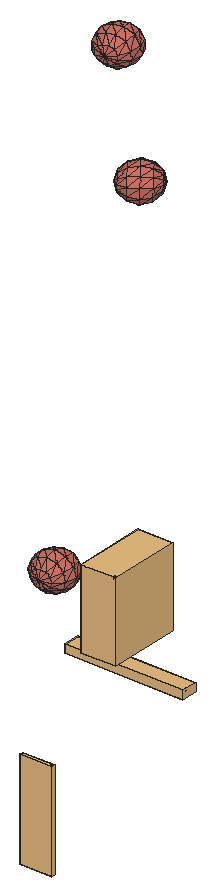
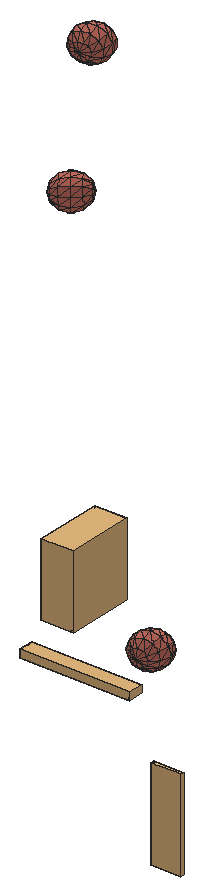
# SketchUp Ruby script. Lengths in inches.
U = 1.inch
M = Sketchup.active_model
def pt(a) = Geom::Point3d.new(a.map { |v| v * U })
def face(e, loops, mat)
  f = e.add_face(loops[0].map { |a| pt(a) })
  loops[1..].each { |l| e.add_face(l.map { |a| pt(a) }).erase! }
  f.material = f.back_material = mat if mat
  f
end
# faces: each face lists its corners as indices into pts; further lists are holes
def faces(e, pts, list, mat = nil) = list.each { |f| face(e, (f[0].is_a?(Array) ? f : [f]).map { |l| l.map { |i| pts[i] } }, mat) }
# xy, xz, yz: faces in a plane at the given z, y or x. An outline is a flat list of corners, or four numbers for a rectangle; further outlines are holes
def ring(l) = l.size == 4 ? [[l[0], l[1]], [l[2], l[1]], [l[2], l[3]], [l[0], l[3]]] : l.each_slice(2).to_a
def flat(e, list, mat, &to3) = list.each { |f| face(e, (f[0].is_a?(Array) ? f : [f]).map { |l| ring(l).map { |u, v| to3.(u, v) } }, mat) }
def xy(e, z, list, mat = nil) = flat(e, list, mat) { |x, y| [x, y, z] }
def xz(e, y, list, mat = nil) = flat(e, list, mat) { |x, z| [x, y, z] }
def yz(e, x, list, mat = nil) = flat(e, list, mat) { |y, z| [x, y, z] }
def lines(e, pts, list) = list.each { |a, b| e.add_line(pt(pts[a]), pt(pts[b])) }
# prism: a flat outline (further loops are holes) pulled along v
def prism(e, loops, v, mat = nil)
  f = face(e, loops, mat); d = Geom::Vector3d.new(v.map { |x| x * U })
  f.pushpull(f.normal.samedirection?(d) ? d.length : -d.length)
end
def box(e, o, s, mat = nil) = prism(e, [[o, [o[0] + s[0], o[1], o[2]], [o[0] + s[0], o[1] + s[1], o[2]], [o[0], o[1] + s[1], o[2]]]], [0, 0, s[2]], mat)
def at(x, y, z, deg = 0) = Geom::Transformation.translation(pt([x, y, z])) * Geom::Transformation.rotation(ORIGIN, Z_AXIS, deg.degrees)
def axes(o, x, y, z) = Geom::Transformation.new([*x, 0, *y, 0, *z, 0, *pt(o).to_a, 1])
def part(name) = M.definitions.add(name)
# library, detail: a bought-in or finely detailed component or shape, given as its bounding box
def library(name, o, s) = part(name).tap { |d| box(d.entities, o, s) }
def detail(e, o, s) = box(e.add_group.entities, o, s)
def put(e, d, t, mat = nil) = e.add_instance(d, t).tap { |i| i.material = mat if mat }
def group(e, t, mat = nil) = e.add_group.tap { |g| g.transformation = t; g.material = mat if mat }.entities
root = M.entities
M.materials.add("green").color = [174, 139, 102]
M.materials.add("vio").color = [206, 114, 100]
c1 = part("3DGeom~226_Defintion")
p = [[20.8,-212.46,-433.01],[-229.2,0,-445.02],[24.02,0,-500],[268.02,-184,-362.99],[268.02,-184,-362.99],[270.8,0,-421],
  [-231.98,184,-387.01],[20.8,212.47,-433.01],[270.8,0,-421],[-231.98,-184,-387.01],[-421,0,-270.8],[-422.61,106.23,-237.31],
  [-422.61,106.23,-237.31],[12.01,-368,-250],[260.4,-318.7,-204.5],[260.4,-318.7,-204.5],[268.02,-184,-362.99],[270.8,0,-421],
  [268.02,184,-362.99],[-239.6,318.7,-228.52],[268.02,184,-362.99],[12.01,368,-250],[-239.6,318.7,-228.52],[12.01,368,-250],
  [443.41,-106.23,-195.7],[268.02,-184,-362.99],[270.8,0,-421],[445.02,0,-229.2],[268.02,184,-362.99],[-239.6,-318.7,-228.52],
  [-239.6,-318.7,-228.52],[-422.61,-106.23,-237.31],[-231.98,-184,-387.01],[-422.61,-106.23,-237.31],[-231.98,184,-387.01],[-422.61,106.23,-237.31],
  [-427.01,184,-145.8],[-231.98,184,-387.01],[-239.6,318.7,-228.52],[439.02,-184,-104.2],[260.4,-318.7,-204.5],[443.41,106.23,-195.7],
  [260.4,318.7,-204.5],[268.02,184,-362.99],[12.01,368,-250],[260.4,318.7,-204.5],[-421,0,-270.8],[-422.61,-106.23,-237.31],
  [-500,0,-24.02],[-421,0,-270.8],[0,-424.93,0],[-239.6,-318.7,-228.52],[12.01,-368,-250],[250,-368,12.01],
  [12.01,-368,-250],[250,-368,12.01],[12.01,-368,-250],[260.4,-318.7,-204.5],[12.01,368,-250],[-239.6,318.7,-228.52],
  [-250,368,-12.01],[260.4,318.7,-204.5],[0,424.93,0],[-239.6,-318.7,-228.52],[-427.01,-184,-145.8],[-422.61,-106.23,-237.31],
  [-422.61,-106.23,-237.31],[500,0,24.02],[-250,-368,-12.01],[-239.6,-318.7,-228.52],[-250,-368,-12.01],[-239.6,-318.7,-228.52],
  [-239.6,318.7,-228.52],[-433.01,212.47,-20.8],[-239.6,318.7,-228.52],[-250,368,-12.01],[433.01,-212.47,20.8],[250,-368,12.01],
  [439.02,184,-104.2],[250,368,12.01],[260.4,318.7,-204.5],[250,368,12.01],[-250,-368,-12.01],[-433.01,-212.46,-20.8],
  [433.01,212.46,20.8],[-439.02,-184,104.2],[-443.41,-106.23,195.7],[-445.02,0,229.2],[-443.41,106.23,195.7],[-439.02,184,104.2],
  [-260.4,-318.7,204.5],[-250,-368,-12.01],[-260.4,-318.7,204.5],[-250,368,-12.01],[-12.01,-368,250],[-260.4,-318.7,204.5],
  [-250,368,-12.01],[-260.4,318.7,204.5],[-260.4,318.7,204.5],[239.6,-318.7,228.52],[239.6,-318.7,228.52],[250,-368,12.01],
  [-260.4,318.7,204.5],[-12.01,368,250],[250,368,12.01],[-12.01,368,250],[427.01,-184,145.8],[239.6,-318.7,228.52],
  [239.6,318.7,228.52],[250,368,12.01],[-12.01,368,250],[239.6,318.7,228.52],[427.01,184,145.8],[422.61,-106.23,237.31],
  [421,0,270.8],[422.61,106.23,237.31],[-268.01,-184,362.99],[-260.4,-318.7,204.5],[-268.01,-184,362.99],[-260.4,318.7,204.5],
  [231.99,184,387.01],[231.99,184,387.01],[-270.8,0,421],[-268.01,-184,362.99],[-270.8,0,421],[-268.01,184,362.99],
  [-260.4,318.7,204.5],[-268.01,184,362.99],[-20.8,-212.47,433.01],[-260.4,-318.7,204.5],[-12.01,-368,250],[-268.01,-184,362.99],
  [-260.4,-318.7,204.5],[-12.01,368,250],[-260.4,318.7,204.5],[-268.01,184,362.99],[231.99,-184,387.01],[-12.01,-368,250],
  [239.6,-318.7,228.52],[231.99,-184,387.01],[239.6,318.7,228.52],[-20.8,212.47,433.01],[231.99,184,387.01],[239.6,318.7,228.52],
  [-268.01,184,362.99],[-270.8,0,421],[421,0,270.8],[231.99,-184,387.01],[422.61,-106.23,237.31],[422.61,106.23,237.31],
  [229.2,0,445.02],[422.61,106.23,237.31],[421,0,270.8],[231.99,-184,387.01],[-12.01,-368,250],[421,0,270.8],
  [231.99,-184,387.01],[-24.02,0,500],[-270.8,0,421],[231.99,-184,387.01]]
faces(c1.entities,p,[[0,1,2],[3,0,2],[4,2,5],[2,1,6],[2,6,7],[8,2,7],[0,9,1],[9,10,1],
  [1,10,11],[1,12,6],[13,9,0],[14,13,0],[15,0,16],[17,7,18],[7,6,19],[20,7,21],
  [7,22,23],[24,25,26],[24,26,27],[27,26,28],[13,29,9],[30,31,32],[9,33,10],[34,35,36],
  [37,36,38],[39,40,25],[39,25,24],[27,28,41],[41,28,42],[43,44,45],[46,47,48],[35,49,48],
  [50,51,52],[53,50,54],[55,56,57],[58,59,60],[61,58,62],[58,60,62],[63,64,65],[66,64,48],
  [36,35,48],[24,27,67],[27,41,67],[50,68,69],[70,64,71],[72,36,73],[74,73,75],[76,77,40],
  [76,40,39],[41,42,78],[78,42,79],[80,62,81],[39,24,67],[41,78,67],[82,83,64],[64,83,48],
  [73,36,48],[76,39,67],[78,84,67],[78,79,84],[83,85,48],[85,86,48],[86,87,48],[87,88,48],
  [88,89,48],[89,73,48],[90,83,91],[92,85,83],[93,73,89],[94,68,50],[94,95,68],[96,89,97],
  [62,60,98],[99,94,50],[100,50,101],[62,102,103],[104,62,105],[106,107,77],[106,77,76],[84,79,108],
  [109,110,111],[106,76,67],[84,112,67],[84,108,112],[113,106,67],[114,113,67],[115,114,67],[112,115,67],
  [116,85,117],[118,86,85],[119,89,88],[113,107,106],[112,120,115],[112,108,121],[122,86,123],[124,87,86],
  [125,88,87],[126,88,127],[128,129,130],[128,131,132],[133,134,135],[136,137,138],[113,139,107],[140,141,142],
  [143,133,141],[144,87,145],[146,147,148],[149,142,150],[151,150,152],[153,128,154],[133,135,141],[155,150,156],
  [157,131,128],[157,158,131],[141,135,158],[150,128,159],[142,141,157],[142,157,150],[141,158,157],[150,157,128]],"vio")
c2 = library("3DGeom~7_Defintion",[-18.22,-500,-162.45],[36.44,1000,324.9])
c3 = part("3DGeom~8_Defintion")
p = [[-16.01,-498.52,-143.51],[-1.98,-500,-151.67],[-15.8,-495.57,-127.57],[-1.98,-500,-151.67],[-16.01,-498.52,-143.51],[-10.11,-499.6,-149.43],
  [-15.8,-495.57,-127.57],[-1.98,-500,-151.67],[-1.57,-494.09,-119.79],[-1.98,-500,-151.67],[6.21,-499.6,-149.64],[12.25,-498.52,-143.88],
  [12.46,-495.57,-127.94],[12.25,-498.52,-143.88],[12.46,-495.57,-127.94],[12.25,-498.52,-143.88],[14.54,-497.04,-135.94],[-16.01,-498.52,-143.51],
  [-15.8,-495.57,-127.57],[-18.09,-497.04,-135.52],[-1.57,-494.09,-119.79],[12.46,-495.57,-127.94],[6.57,-494.49,-122.03],[-15.8,-495.57,-127.57],
  [-1.57,-494.09,-119.79],[-9.75,-494.49,-121.82],[1.71,500,131.72],[-6.08,491.3,160.5],[2.11,490.68,162.45],[1.71,500,131.72],
  [2.11,490.68,162.45],[10.24,491.3,160.28],[1.71,500,131.72],[-12.12,493.01,154.95],[-6.08,491.3,160.5],[1.71,500,131.72],
  [10.24,491.3,160.28],[16.14,493.01,154.58],[1.71,500,131.72],[-14.41,495.34,147.3],[-12.12,493.01,154.95],[1.71,500,131.72],
  [16.14,493.01,154.58],[18.22,495.34,146.87],[1.71,500,131.72],[-12.32,497.67,139.58],[-14.41,495.34,147.3],[1.71,500,131.72],
  [18.22,495.34,146.87],[15.9375,497.67,139.22],[1.71,500,131.72],[-6.42,499.375,133.88],[-12.32,497.67,139.58],[1.71,500,131.72],
  [15.9375,497.67,139.22],[9.89,499.375,133.67]]
faces(c3.entities,p,[[0,1,2],[3,4,5],[6,7,8],[9,10,11],[12,7,13],[8,7,12],[14,15,16],[17,18,19],
  [20,21,22],[23,24,25],[26,27,28],[29,30,31],[32,33,34],[35,36,37],[38,39,40],[41,42,43],
  [44,45,46],[47,48,49],[50,51,52],[53,54,55]],"green")
c4 = library("3DGeom~117_Defintion",[-67.35,-35.15,-500],[134.7,70.3,1000])
c5 = part("3DGeom~118_Defintion")
p = [[-32.48,-34.33,-497.04],[-40.08,-25.16,-500],[-19.94,-32.92,-492.22],[-40.08,-25.16,-500],[-32.48,-34.33,-497.04],[-37.63,-30.67,-499.04],
  [-19.94,-32.92,-492.22],[-40.08,-25.16,-500],[-15,-22.34,-490.36],[-40.08,-25.16,-500],[-39.16,-19.27,-499.67],[-35.13,-14.58,-498.14],
  [-22.6,-13.17,-493.32],[-40.08,-25.16,-500],[-35.13,-14.58,-498.14],[-15,-22.34,-490.36],[-40.08,-25.16,-500],[-22.6,-13.17,-493.32],
  [-22.6,-13.17,-493.32],[-35.13,-14.58,-498.14],[-29.07,-12.35,-495.8125],[-32.48,-34.33,-497.04],[-19.94,-32.92,-492.22],[-26.01,-35.15,-494.55],
  [-15,-22.34,-490.36],[-22.6,-13.17,-493.32],[-17.45,-16.83,-491.32],[-19.94,-32.92,-492.22],[-15,-22.34,-490.36],[-15.92,-28.23,-490.69],
  [40.93,22.57,500],[66.34,19.07,495.46],[67.35,24.92,494.8],[40.93,22.57,500],[64.81,30.47,494.83],[59.41,34.21,495.55],
  [40.93,22.57,500],[67.35,24.92,494.8],[64.81,30.47,494.83],[40.93,22.57,500],[62.07,14.46,496.64],[66.34,19.07,495.46],
  [40.93,22.57,500],[59.41,34.21,495.55],[52.61,35.15,496.77],[40.93,22.57,500],[55.67,12.35,498.03],[62.07,14.46,496.64],
  [40.93,22.57,500],[52.61,35.15,496.77],[46.21,33.04,498.15],[40.93,22.57,500],[48.86,13.29,499.25],[55.67,12.35,498.03],
  [40.93,22.57,500],[46.21,33.04,498.15],[41.93,28.43,499.34],[40.93,22.57,500],[43.47,17.03,499.97],[48.86,13.29,499.25]]
faces(c5.entities,p,[[0,1,2],[3,4,5],[6,7,8],[9,10,11],[12,13,14],[15,16,17],[18,19,20],[21,22,23],
  [24,25,26],[27,28,29],[30,31,32],[33,34,35],[36,37,38],[39,40,41],[42,43,44],[45,46,47],
  [48,49,50],[51,52,53],[54,55,56],[57,58,59]],"green")
c6 = library("3DGeom~115_Defintion",[-457.23,-500,-223.02],[914.46,1000,446.04])
c7 = part("3DGeom~116_Defintion")
p = [[-442.89,-492.22,-212.42],[-434.63,-497.16,-209.35],[-428.12,-500,-201.74],[-426.4,-497.09,-181.7],[-442.89,-492.22,-212.42],[-428.12,-500,-201.74],
  [-439.45,-486.4,-172.35],[-442.89,-492.22,-212.42],[-426.4,-497.09,-181.7],[-455.93,-481.53,-203.07],[-442.89,-492.22,-212.42],[-454.21,-478.62,-183.03],
  [-442.89,-492.22,-212.42],[-455.93,-481.53,-203.07],[-450.6875,-486.5,-210.125],[-454.21,-478.62,-183.03],[-442.89,-492.22,-212.42],[-439.45,-486.4,-172.35],
  [-455.93,-481.53,-203.07],[-454.21,-478.62,-183.03],[-457.23,-478.65,-193.16],[-426.4,-497.09,-181.7],[-428.12,-500,-201.74],[-425.11,-499.97,-191.61],
  [-454.21,-478.62,-183.03],[-439.45,-486.4,-172.35],[-447.71,-481.46,-175.42],[-439.45,-486.4,-172.35],[-426.4,-497.09,-181.7],[-431.65,-492.12,-174.65],
  [445.89,493.0625,185.04],[444.32,479.16,220.86],[452.08,476.9375,214.19],[445.89,493.0625,185.04],[452.08,476.9375,214.19],[456.81,477.81,204.8],
  [445.89,493.0625,185.04],[456.81,477.81,204.8],[457.23,481.53,195.2],[445.89,493.0625,185.04],[435.6,483.875,223.02],[444.32,479.16,220.86],
  [445.89,493.0625,185.04],[457.23,481.53,195.2],[453.23,487.12,187.97],[445.89,493.0625,185.04],[428.26,489.82,220.09],[435.6,483.875,223.02],
  [445.89,493.0625,185.04],[424.27,495.41,212.85],[428.26,489.82,220.09],[445.89,493.0625,185.04],[424.6875,499.13,203.26],[424.27,495.41,212.85],
  [445.89,493.0625,185.04],[429.41,500,193.87],[424.6875,499.13,203.26],[445.89,493.0625,185.04],[437.17,497.78,187.2],[429.41,500,193.87]]
faces(c7.entities,p,[[0,1,2],[3,4,5],[6,7,8],[9,10,11],[12,13,14],[15,16,17],[18,19,20],[21,22,23],
  [24,25,26],[27,28,29],[30,31,32],[33,34,35],[36,37,38],[39,40,41],[42,43,44],[45,46,47],
  [48,49,50],[51,52,53],[54,55,56],[57,58,59]],"green")
c8 = part("3DGeom~198_Defintion")
p = [[-186.75,95.89,-455.78],[73.04,104.68,-484.59],[66.15,-117.28,-481.5625],[307.29,-106.8,-380.93],[313.25,85.42,-383.56],[60.35,298.59,-357.77],
  [-197.73,263.82,-345.95],[-192.71,-96.34,-453.16],[41.54,-307.82,-349.5],[285.98,-271.8125,-266.57],[-396.49,61.4,-304.84],[-402.84,158.36,-241.43],
  [-396.49,61.4,-304.84],[-402.84,158.36,-241.43],[-214.02,-261.34,-338.79],[-399.9375,-49.58,-303.33],[-396.49,61.4,-304.84],[-399.9375,-49.58,-303.33],
  [313.25,85.42,-383.56],[466.09,-67.71,-178.23],[307.29,-106.8,-380.93],[313.25,85.42,-383.56],[469.53,43.27,-179.75],[302.27,253.36,-273.73],
  [313.25,85.42,-383.56],[302.27,253.36,-273.73],[307.29,-106.8,-380.93],[453.78,-162.97,-112.2],[285.98,-271.8125,-266.57],[307.29,-106.8,-380.93],
  [31.5,412.5,-135.08],[302.27,253.36,-273.73],[60.35,298.59,-357.77],[-222.72,362.47,-153.1],[60.35,298.59,-357.77],[-197.73,263.82,-345.95],
  [-222.72,362.47,-153.1],[60.35,298.59,-357.77],[-214.02,-261.34,-338.79],[41.54,-307.82,-349.5],[5.8,-415.875,-123.8],[41.54,-307.82,-349.5],
  [255.02,-365.39,-71.1],[41.54,-307.82,-349.5],[285.98,-271.8125,-266.57],[-417.26,215.3125,-130.09],[-197.73,263.82,-345.95],[-402.84,158.36,-241.43],
  [-222.72,362.47,-153.1],[-197.73,263.82,-345.95],[-214.02,-261.34,-338.79],[-244.98,-354.93,-143.32],[-412.24,-144.85,-237.3],[-214.02,-261.34,-338.79],
  [-244.98,-354.93,-143.32],[-399.9375,-49.58,-303.33],[-412.24,-144.85,-237.3],[-396.49,61.4,-304.84],[-399.9375,-49.58,-303.33],[-500,10.47,-72.22],
  [302.27,253.36,-273.73],[463.1875,140.23,-116.34],[277.28,352,-80.875],[302.27,253.36,-273.73],[277.28,352,-80.875],[302.27,253.36,-273.73],
  [285.98,-271.8125,-266.57],[435.91,-217,0.65],[255.02,-365.39,-71.1],[285.98,-271.8125,-266.57],[-430.11,-198.87,-124.44],[500,-10.47,72.22],
  [-435.91,217,-0.65],[-255.02,365.39,71.1],[-255.02,365.39,71.1],[-222.72,362.47,-153.1],[-244.98,-354.93,-143.32],[-31.5,-412.49,135.08],
  [-244.98,-354.93,-143.32],[-277.28,-352,80.875],[-277.28,-352,80.875],[-5.8,415.875,123.8],[-255.02,365.39,71.1],[-448.76,-197.18,5],
  [222.72,-362.47,153.1],[448.76,197.18,-4.99],[277.28,352,-80.875],[244.98,354.93,143.32],[277.28,352,-80.875],[244.98,354.93,143.32],
  [-463.1875,-140.23,116.34],[-469.53,-43.27,179.75],[-466.09,67.71,178.23],[-453.78,162.97,112.2],[255.02,-365.39,-71.1],[417.26,-215.3125,130.09],
  [222.72,-362.47,153.1],[255.02,-365.39,-71.1],[430.11,198.87,124.44],[244.98,354.93,143.32],[-302.27,-253.36,273.73],[-285.98,271.8125,266.57],
  [-285.98,271.8125,266.57],[-255.02,365.39,71.1],[402.84,-158.36,241.43],[396.49,-61.4,304.84],[402.84,-158.36,241.43],[399.9375,49.58,303.33],
  [396.49,-61.4,304.84],[412.24,144.85,237.3],[399.9375,49.58,303.33],[-277.28,-352,80.875],[-60.35,-298.59,357.77],[-277.28,-352,80.875],
  [-60.35,-298.59,357.77],[-302.27,-253.36,273.73],[-313.25,-85.42,383.56],[-285.98,271.8125,266.57],[-41.54,307.82,349.5],[214.02,261.34,338.79],
  [214.02,261.34,338.79],[244.98,354.93,143.32],[222.72,-362.47,153.1],[402.84,-158.36,241.43],[197.73,-263.82,345.95],[-60.35,-298.59,357.77],
  [197.73,-263.82,345.95],[214.02,261.34,338.79],[222.72,-362.47,153.1],[402.84,-158.36,241.43],[197.73,-263.82,345.95],[-307.29,106.8,380.93],
  [192.71,96.34,453.16],[399.9375,49.58,303.33],[412.24,144.85,237.3],[412.24,144.85,237.3],[214.02,261.34,338.79],[197.73,-263.82,345.95],
  [402.84,-158.36,241.43],[396.49,-61.4,304.84],[-307.29,106.8,380.93],[-41.54,307.82,349.5],[-285.98,271.8125,266.57],[-302.27,-253.36,273.73],
  [-60.35,-298.59,357.77],[-73.04,-104.68,484.59],[-302.27,-253.36,273.73],[-313.25,-85.42,383.56],[186.75,-95.89,455.78],[-66.15,117.28,481.5625],
  [214.02,261.34,338.79],[214.02,261.34,338.79],[-41.54,307.82,349.5],[-307.29,106.8,380.93],[-41.54,307.82,349.5],[-313.25,-85.42,383.56],
  [-307.29,106.8,380.93],[-313.25,-85.42,383.56]]
faces(c8.entities,p,[[0,1,2],[1,3,2],[1,4,3],[5,4,1],[6,1,0],[6,5,1],[7,2,8],[2,9,8],
  [2,3,9],[0,2,7],[10,0,7],[11,0,12],[13,6,0],[7,8,14],[15,7,14],[16,7,17],
  [18,19,20],[21,22,19],[23,22,24],[5,25,4],[26,27,28],[29,19,27],[30,31,32],[33,34,35],
  [36,30,37],[38,39,40],[41,42,40],[43,44,42],[45,46,47],[45,48,49],[50,40,51],[52,53,54],
  [55,14,56],[57,58,59],[47,57,59],[58,52,59],[60,61,22],[62,61,63],[30,64,65],[66,67,68],
  [69,27,67],[45,47,59],[52,54,70],[52,70,59],[19,22,71],[22,61,71],[27,19,71],[72,48,45],
  [72,73,48],[74,30,75],[76,40,77],[78,77,79],[70,54,80],[81,64,30],[82,81,30],[72,45,59],
  [70,80,83],[70,83,59],[40,84,77],[40,42,84],[61,85,71],[86,85,61],[67,27,71],[87,85,88],
  [81,89,64],[83,90,59],[90,91,59],[91,92,59],[93,72,59],[92,93,59],[94,95,96],[97,67,95],
  [85,98,71],[99,98,85],[93,73,72],[95,67,71],[83,80,100],[83,100,90],[93,101,73],[102,81,103],
  [104,95,71],[105,106,71],[107,108,71],[109,110,71],[98,109,71],[111,77,112],[113,114,115],[92,101,93],
  [90,100,116],[90,116,91],[117,118,81],[118,89,81],[119,109,98],[120,98,121],[122,95,123],[77,124,125],
  [77,84,126],[118,127,89],[128,129,130],[91,131,92],[92,131,101],[91,116,131],[132,133,134],[132,135,136],
  [137,138,139],[140,141,142],[143,144,145],[146,145,147],[148,139,133],[148,133,132],[137,139,148],[149,132,150],
  [149,151,152],[144,137,148],[153,149,154],[144,148,145],[155,149,156],[157,145,149],[145,148,132],[145,132,149]],"vio")
c9 = part("3DGeom~197_Defintion")
p = [[121.86,-140.79,-463.73],[-185.76,-85.76,-461.18],[69.15,-43.45,-500],[305.53,10.51,-404.84],[-186.34,107.23,-454.67],[68.81,67.97,-496.24],
  [305.53,10.51,-404.84],[120.9375,163.62,-453.46],[305.53,10.51,-404.84],[-96.06,272.89,-380.57],[-94.47,-254.36,-398.36],[212.81,-197.97,-397.15],
  [305.53,10.51,-404.84],[-390.89,-105.1,-298.79],[-391.57,117.75,-291.27],[-287.32,309.04,-205.7],[-287.32,309.04,-205.7],[211.56,217.86,-383.12],
  [305.53,10.51,-404.84],[60.9,366.84,-258.73],[60.9,366.84,-258.73],[317.64,-199.66,-318.1],[305.53,10.51,-404.84],[408.26,-145.42,-247.75],
  [305.53,10.51,-404.84],[460.38,-49.77,-204.97],[408.26,-145.42,-247.75],[305.53,10.51,-404.84],[460.04,61.65,-201.21],[316.39,216.17,-304.0625],
  [305.53,10.51,-404.84],[407.34,158.99,-237.48],[316.39,216.17,-304.0625],[63.06,-353.4,-283.04],[-285.48,-299.78,-226.25],[-94.47,-254.36,-398.36],
  [63.06,-353.4,-283.04],[-285.48,-299.78,-226.25],[317.64,-199.66,-318.1],[63.06,-353.4,-283.04],[212.81,-197.97,-397.15],[211.56,217.86,-383.12],
  [242.47,363.91,-121.81],[316.39,216.17,-304.0625],[211.56,217.86,-383.12],[60.9,366.84,-258.73],[242.47,363.91,-121.81],[-96.06,272.89,-380.57],
  [-287.32,309.04,-205.7],[-106.08,417.53,-65.02],[-96.06,272.89,-380.57],[317.64,-199.66,-318.1],[244.64,-356.33,-146.11],[63.06,-353.4,-283.04],
  [244.64,-356.33,-146.11],[317.64,-199.66,-318.1],[400,264.87,-6.48],[242.47,363.91,-121.81],[-285.48,-299.78,-226.25],[-491.29,-96.27,-56.34],
  [-390.89,-105.1,-298.79],[-390.89,-105.1,-298.79],[-491.87,96.72,-49.82],[-390.89,-105.1,-298.79],[-391.57,117.75,-291.27],[-391.57,117.75,-291.27],
  [-401.59,262.38,24.28],[-391.57,117.75,-291.27],[-401.59,262.38,24.28],[-287.32,309.04,-205.7],[63.06,-353.4,-283.04],[-103.58,-414.14,-93.09],
  [-285.48,-299.78,-226.25],[63.06,-353.4,-283.04],[103.58,414.14,93.09],[242.47,363.91,-121.81],[401.59,-262.38,-24.28],[244.64,-356.33,-146.11],
  [491.29,96.27,56.34],[-400,-264.87,6.48],[-285.48,-299.78,-226.25],[-285.48,-299.78,-226.25],[-400,-264.87,6.48],[-401.59,262.38,24.28],
  [-244.64,356.33,146.11],[491.87,-96.72,49.82],[106.08,-417.53,65.02],[401.59,-262.38,-24.28],[242.47,363.91,-121.81],[285.48,299.78,226.25],
  [400,264.87,-6.48],[242.47,363.91,-121.81],[285.48,299.78,226.25],[-242.47,-363.91,121.81],[-400,-264.87,6.48],[-63.06,353.4,283.04],
  [-460.04,-61.65,201.21],[-460.38,49.77,204.97],[-408.26,145.42,247.75],[-401.59,262.38,24.28],[401.59,-262.38,-24.28],[287.32,-309.04,205.7],
  [287.32,-309.04,205.7],[390.89,105.1,298.79],[285.48,299.78,226.25],[-242.47,-363.91,121.81],[-407.34,-158.99,237.48],[-401.59,262.38,24.28],
  [-317.64,199.66,318.1],[-401.59,262.38,24.28],[-317.64,199.66,318.1],[-244.64,356.33,146.11],[391.57,-117.75,291.27],[-60.9,-366.84,258.73],
  [287.32,-309.04,205.7],[94.47,254.36,398.36],[94.47,254.36,398.36],[285.48,299.78,226.25],[-316.39,-216.17,304.0625],[-242.47,-363.91,121.81],
  [-316.39,-216.17,304.0625],[-317.64,199.66,318.1],[-212.81,197.97,397.15],[-212.81,197.97,397.15],[-305.53,-10.51,404.84],[-305.53,-10.51,404.84],
  [-305.53,-10.51,404.84],[287.32,-309.04,205.7],[96.06,-272.89,380.57],[391.57,-117.75,291.27],[96.06,-272.89,380.57],[287.32,-309.04,205.7],
  [285.48,299.78,226.25],[94.47,254.36,398.36],[185.76,85.76,461.18],[285.48,299.78,226.25],[390.89,105.1,298.79],[-305.53,-10.51,404.84],
  [-317.64,199.66,318.1],[-408.26,145.42,247.75],[-305.53,-10.51,404.84],[-211.56,-217.86,383.11],[-316.39,-216.17,304.0625],[-211.56,-217.86,383.11],
  [-60.9,-366.84,258.73],[-63.06,353.4,283.04],[-212.81,197.97,397.15],[-121.86,140.79,463.73],[-63.06,353.4,283.04],[391.57,-117.75,291.27],
  [186.34,-107.23,454.67],[390.89,105.1,298.79],[391.57,-117.75,291.27],[390.89,105.1,298.79],[-316.39,-216.17,304.0625],[-211.56,-217.86,383.11],
  [-317.64,199.66,318.1],[-120.9375,-163.62,453.46],[-211.56,-217.86,383.11],[-211.56,-217.86,383.11],[-69.15,43.45,500],[-68.81,-67.97,496.24]]
faces(c9.entities,p,[[0,1,2],[0,2,3],[2,1,4],[2,4,5],[2,5,6],[5,7,8],[5,4,9],[5,9,7],
  [0,10,1],[11,10,0],[11,0,12],[10,13,1],[1,13,14],[1,14,4],[4,14,15],[4,16,9],
  [7,17,18],[7,9,19],[7,20,17],[21,11,22],[23,21,24],[25,26,27],[28,25,27],[17,29,30],
  [31,28,27],[32,31,27],[33,34,35],[11,36,10],[10,37,13],[38,39,40],[41,42,43],[44,45,46],
  [47,48,49],[50,49,45],[51,52,53],[26,54,55],[32,56,31],[32,57,56],[58,59,60],[61,59,62],
  [63,62,64],[65,62,66],[67,68,69],[70,71,72],[52,71,73],[45,74,75],[45,49,74],[26,76,77],
  [25,76,26],[31,78,28],[31,56,78],[71,79,80],[81,82,59],[48,83,84],[48,84,49],[25,85,76],
  [28,85,25],[28,78,85],[52,86,71],[87,86,52],[88,89,90],[91,74,92],[86,93,71],[71,93,94],
  [49,84,95],[49,95,74],[82,96,59],[59,97,62],[59,96,97],[62,97,98],[62,98,99],[100,101,86],
  [85,102,76],[56,103,78],[56,104,103],[105,106,82],[82,106,96],[107,98,108],[109,110,111],[85,112,102],
  [78,112,85],[78,103,112],[86,113,93],[114,113,86],[74,95,115],[74,116,117],[113,118,93],[119,120,106],
  [84,121,122],[84,123,95],[96,106,124],[97,96,125],[98,97,126],[127,128,113],[129,130,131],[132,133,134],
  [135,134,136],[106,120,137],[138,139,140],[113,141,142],[130,143,144],[145,146,147],[148,147,133],[149,150,130],
  [151,150,152],[153,134,150],[154,155,140],[146,156,140],[130,157,158],[150,157,130],[159,157,140],[147,146,140],
  [133,147,160],[133,160,134],[157,161,140],[161,160,140],[160,147,140],[150,161,157],[134,161,150],[134,160,161]],"vio")
g1 = group(root,at(15.3125,38.42,26.21))
put(g1,c1,axes([2.27,0.57,12.375],[0,0.00039,0],[0,0,-0.00039],[-0.00039,0,0]),"vio")
g2 = group(root,at(15.3125,38.42,26.21))
put(g2,c2,axes([2.46,0.13,10.61],[0,0.00091,0],[0,0,-0.00091],[-0.00091,0,0]),"green")
put(g2,c3,axes([2.46,0.13,10.61],[0,0.00091,0],[0,0,-0.00091],[-0.00091,0,0]),"green")
g3 = group(root,at(15.3125,38.42,26.21))
put(g3,c4,axes([3.04,0.48,11.875],[0,0.00109,0],[0,0,-0.00109],[-0.00109,0,0]),"green")
put(g3,c5,axes([3.04,0.48,11.875],[0,0.00109,0],[0,0,-0.00109],[-0.00109,0,0]),"green")
g4 = group(root,at(15.3125,38.42,26.21))
put(g4,c6,axes([3.2,0.24,12.62],[0,0.00073,0],[0,0,-0.00073],[-0.00073,0,0]),"green")
put(g4,c7,axes([3.2,0.24,12.62],[0,0.00073,0],[0,0,-0.00073],[-0.00073,0,0]),"green")
g5 = group(root,at(15.3125,38.42,26.21))
put(g5,c8,axes([3.21,0.13,17.26],[0,0.00039,0],[0,0,-0.00039],[-0.00039,0,0]),"vio")
g6 = group(root,at(15.3125,38.42,26.21))
put(g6,c9,axes([3.23,0.36,16.03],[0,0.00038,0],[0,0,-0.00038],[-0.00038,0,0]),"vio")
